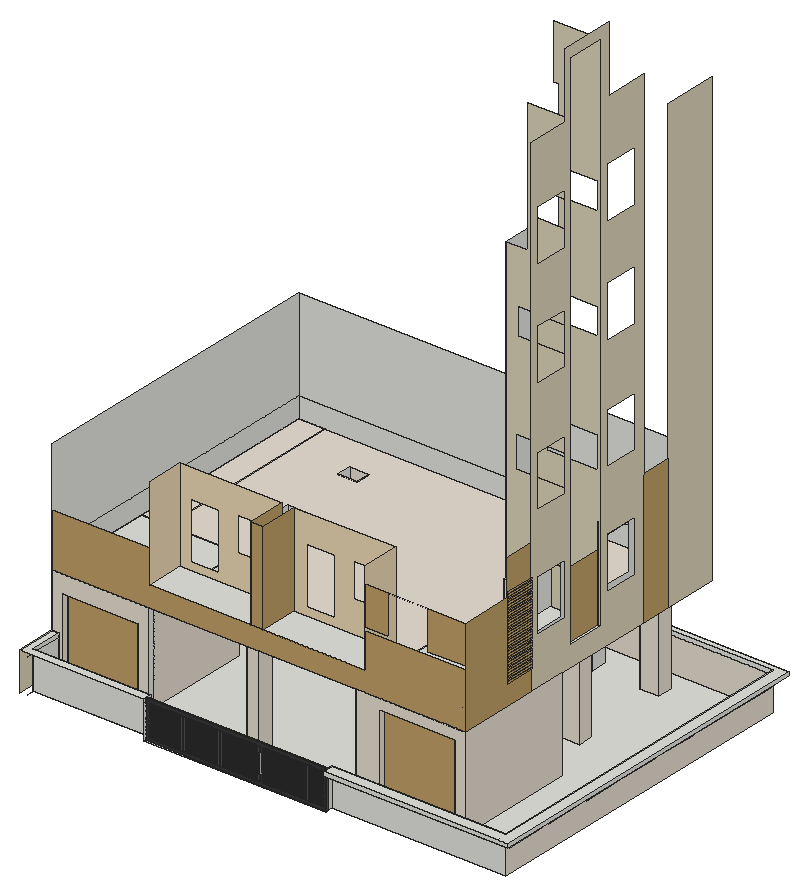
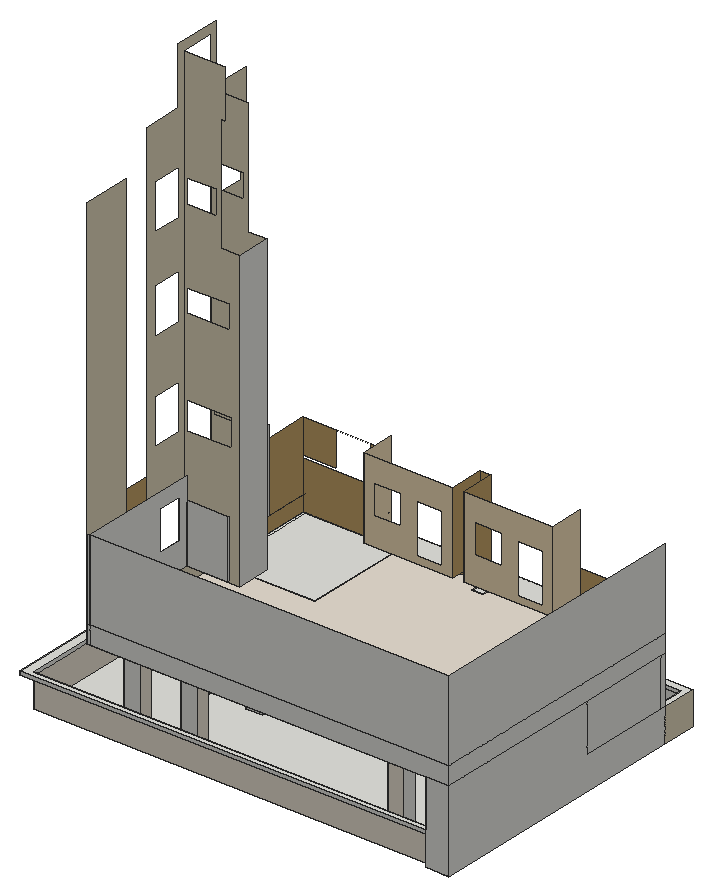
# SketchUp Ruby script. Lengths in inches.
U = 1.inch
M = Sketchup.active_model
def pt(a) = Geom::Point3d.new(a.map { |v| v * U })
def face(e, loops, mat)
  f = e.add_face(loops[0].map { |a| pt(a) })
  loops[1..].each { |l| e.add_face(l.map { |a| pt(a) }).erase! }
  f.material = f.back_material = mat if mat
  f
end
# faces: each face lists its corners as indices into pts; further lists are holes
def faces(e, pts, list, mat = nil) = list.each { |f| face(e, (f[0].is_a?(Array) ? f : [f]).map { |l| l.map { |i| pts[i] } }, mat) }
# xy, xz, yz: faces in a plane at the given z, y or x. An outline is a flat list of corners, or four numbers for a rectangle; further outlines are holes
def ring(l) = l.size == 4 ? [[l[0], l[1]], [l[2], l[1]], [l[2], l[3]], [l[0], l[3]]] : l.each_slice(2).to_a
def flat(e, list, mat, &to3) = list.each { |f| face(e, (f[0].is_a?(Array) ? f : [f]).map { |l| ring(l).map { |u, v| to3.(u, v) } }, mat) }
def xy(e, z, list, mat = nil) = flat(e, list, mat) { |x, y| [x, y, z] }
def xz(e, y, list, mat = nil) = flat(e, list, mat) { |x, z| [x, y, z] }
def yz(e, x, list, mat = nil) = flat(e, list, mat) { |y, z| [x, y, z] }
def lines(e, pts, list) = list.each { |a, b| e.add_line(pt(pts[a]), pt(pts[b])) }
# prism: a flat outline (further loops are holes) pulled along v
def prism(e, loops, v, mat = nil)
  f = face(e, loops, mat); d = Geom::Vector3d.new(v.map { |x| x * U })
  f.pushpull(f.normal.samedirection?(d) ? d.length : -d.length)
end
def box(e, o, s, mat = nil) = prism(e, [[o, [o[0] + s[0], o[1], o[2]], [o[0] + s[0], o[1] + s[1], o[2]], [o[0], o[1] + s[1], o[2]]]], [0, 0, s[2]], mat)
def at(x, y, z, deg = 0) = Geom::Transformation.translation(pt([x, y, z])) * Geom::Transformation.rotation(ORIGIN, Z_AXIS, deg.degrees)
def axes(o, x, y, z) = Geom::Transformation.new([*x, 0, *y, 0, *z, 0, *pt(o).to_a, 1])
def part(name) = M.definitions.add(name)
# library, detail: a bought-in or finely detailed component or shape, given as its bounding box
def library(name, o, s) = part(name).tap { |d| box(d.entities, o, s) }
def detail(e, o, s) = box(e.add_group.entities, o, s)
def put(e, d, t, mat = nil) = e.add_instance(d, t).tap { |i| i.material = mat if mat }
def group(e, t, mat = nil) = e.add_group.tap { |g| g.transformation = t; g.material = mat if mat }.entities
root = M.entities
M.materials.add("Generic").color = [191, 159, 103]
M.materials.add("Generic\#2").color = [235, 215, 180]
M.materials.add("Generic\#3").color = [218, 209, 183]
M.materials.add("Generic\#5").color = [230, 221, 208]
M.materials.add("[Color M02]").color = [198, 198, 198]
M.materials.add("[Color M06]").color = [86, 86, 86]
M.materials.add("[Color M07]").color = [58, 58, 58]
c1 = part("Group\#5")
xy(c1.entities,0,[[0,0,1,57.75]])
xy(c1.entities,2.57,[[0,0,1,57.75]])
xz(c1.entities,0,[[0,0,1,2.57]])
xz(c1.entities,57.75,[[0,0,1,2.57]])
yz(c1.entities,1,[[0,0,57.75,2.57]])
c2 = part("Group\#6")
put(c2.entities,c1,at(0,0,4.75))
put(c2.entities,c1,at(0,0,0))
put(c2.entities,c1,at(0,0,19))
put(c2.entities,c1,at(0,0,28.5))
put(c2.entities,c1,at(0,0,133))
put(c2.entities,c1,at(0,0,152))
put(c2.entities,c1,at(0,0,128.25))
put(c2.entities,c1,at(0,0,9.5))
put(c2.entities,c1,at(0,0,123.5))
put(c2.entities,c1,at(0,0,114))
put(c2.entities,c1,at(0,0,147.25))
put(c2.entities,c1,at(0,0,118.75))
put(c2.entities,c1,at(0,0,142.5))
put(c2.entities,c1,at(0,0,109.25))
put(c2.entities,c1,at(0,0,137.75))
put(c2.entities,c1,at(0,0,104.5))
put(c2.entities,c1,at(0,0,99.75))
put(c2.entities,c1,at(0,0,95))
put(c2.entities,c1,at(0,0,85.5))
put(c2.entities,c1,at(0,0,80.75))
put(c2.entities,c1,at(0,0,90.25))
put(c2.entities,c1,at(0,0,76))
put(c2.entities,c1,at(0,0,71.25))
put(c2.entities,c1,at(0,0,38))
put(c2.entities,c1,at(0,0,14.25))
put(c2.entities,c1,at(0,0,33.25))
put(c2.entities,c1,at(0,0,57))
put(c2.entities,c1,at(0,0,23.75))
put(c2.entities,c1,at(0,0,61.75))
put(c2.entities,c1,at(0,0,156.75))
put(c2.entities,c1,at(0,0,47.5))
put(c2.entities,c1,at(0,0,52.25))
put(c2.entities,c1,at(0,0,42.75))
put(c2.entities,c1,at(0,0,66.5))
xy(root,0,[[245.8125,5.75,599.47,21.4375],[[17.8125,21.4375,937.125,21.4375,937.125,671.4375,55.33,671.4375,55.33,683.8125,4.1875,683.8125,4.1875,83.8125,17.8125,83.8125],[596.08,83.8125,596.08,317.4375,809.375,317.4375,809.375,83.8125,787.75,83.8125,787.75,94.5625,641.71,94.5625,641.71,83.8125],[171.85,83.8125,193.48,301.3125],[17.8125,83.8125,25.82,301.3125],[159.02,434.88,196.46,463.32],[159.02,585.95,196.46,614.38],[613.85,411.28,651.29,439.72],[604.67,603.65,642.1,632.09],[731.98,603.65,769.42,632.09],[731.98,411.28,769.42,439.72],[382.78,83.8125,406.78,116.4375]],[17.8125,83.8125,25.82,94.5625],[171.85,83.8125,193.48,94.5625],[382.78,83.8125,406.78,116.4375],
  [596.08,83.8125,641.71,83.8125,641.71,94.5625,787.75,94.5625,787.75,83.8125,809.375,83.8125,809.375,317.4375,596.08,317.4375],[17.8125,94.5625,25.82,301.3125],[171.85,94.5625,193.48,301.3125]])
xy(root,59.89,[[950.0625,12.05,952.875,89.02],[950.0625,107.24,952.875,180.9],[950.0625,199.12,952.875,272.77],[950.0625,290.99,952.875,364.65],[950.0625,382.87,952.875,456.52],
  [950.0625,474.74,952.875,548.4],[950.0625,566.62,952.875,640.27]],"Generic")
xy(root,66.1875,[[599.47,0,952.875,5.75],[952.875,0,958.625,95.32],[937.125,5.75,937.125,671.4375,55.33,671.4375,55.33,683.8125,952.875,683.8125,952.875,5.75],[952.875,95.32,958.625,100.94],[952.875,100.94,958.625,187.19],
  [952.875,187.19,958.625,192.82],[952.875,192.82,958.625,279.07],[952.875,279.07,958.625,284.69],[952.875,284.69,958.625,370.94],[952.875,370.94,958.625,376.57],
  [952.875,376.57,958.625,462.82],[952.875,462.82,958.625,468.44],[952.875,468.44,958.625,554.69],[952.875,554.69,958.625,560.32],[952.875,560.32,958.625,646.57],
  [952.875,646.57,958.625,652.19],[952.875,652.19,958.625,683.8125]])
xy(root,74,[[599.47,0,958.625,0,958.625,683.8125,55.33,683.8125,55.33,671.4375,937.125,671.4375,937.125,21.4375,599.47,21.4375],[4.1875,5.75,245.8125,5.75,245.8125,21.4375,17.8125,21.4375,17.8125,83.8125,4.1875,83.8125],[4.1875,83.8125,17.8125,94.5625],[4.1875,94.5625,17.8125,301.3125]])
xy(root,144.62,[[25.82,94.5625,171.85,301.3125]])
xy(root,144.62,[[25.82,83.8125,171.85,94.5625]],"Generic\#5")
xy(root,158.37,[[641.71,83.8125,787.75,94.5625]],"Generic\#5")
xy(root,180,[[4.1875,83.8125,193.48,94.5625],[382.78,83.8125,406.78,116.4375],[596.08,83.8125,802.875,317.4375],[802.875,83.8125,809.375,317.4375],[4.1875,94.5625,193.48,301.3125]])
xy(root,180,[[[193.48,83.8125,193.48,301.3125,4.1875,301.3125,4.1875,683.8125,809.375,683.8125,809.375,317.4375,596.08,317.4375,596.08,83.8125,406.78,83.8125,406.78,116.4375,382.78,116.4375,382.78,83.8125],[604.67,603.65,642.1,632.09],[731.98,603.65,769.42,632.09],[613.85,411.28,651.29,439.72],[159.02,434.88,196.46,463.32],[159.02,585.95,196.46,614.38],[731.98,411.28,769.42,439.72]]],"Generic\#5")
xy(root,219.75,[[193.83,83.8125,391.53,158.75],[415.53,83.8125,613.23,158.75],[802.875,185.01,809.375,242.76],[684.5625,338.625,710.73,413.6875],[710.73,338.625,802.875,413.6875],
  [802.875,338.625,809.375,413.6875],[710.73,413.6875,802.875,414.4375]])
xz(root,0,[[599.47,66.1875,958.625,74]])
xz(root,21.4375,[[17.8125,0,245.8125,66.1875],[599.47,0,937.125,66.1875],[17.8125,66.1875,245.8125,74],[599.47,66.1875,937.125,74]])
xz(root,83.8125,[[4.1875,0,17.8125,74]])
xz(root,83.8125,[[4.1875,180,809.375,180,809.375,287.13,613.73,287.13,613.73,294.19,658.76,294.19,658.76,368.44,736.32,368.44,736.32,294.19,809.375,294.19,809.375,368.76,613.23,368.76,613.23,219.75,193.83,219.75,193.83,284.38,4.1875,284.38],[391.53,219.75,415.53,399.75]],"Generic")
xz(root,83.8125,[[17.8125,0,25.82,0,25.82,144.62,171.85,144.62,171.85,0,193.48,0,193.48,180,4.1875,180,4.1875,74,17.8125,74],[382.78,0,406.78,180],[596.08,0,641.71,0,641.71,158.37,787.75,158.37,787.75,0,809.375,0,809.375,180,596.08,180]],"Generic\#5")
xz(root,94.5625,[[17.8125,0,25.82,0,25.82,144.62,171.85,144.62,171.85,0,193.48,0,193.48,180,4.1875,180,4.1875,74,17.8125,74]])
xz(root,94.5625,[[25.82,0,171.85,144.62],[641.71,0,787.75,158.37]],"Generic")
xz(root,116.4375,[[382.78,0,406.78,180]])
xz(root,158.75,[[[193.83,219.75,391.53,399.75],[214.375,234.72,270.0625,344.97],[306.72,282.21,366.62,348.04]],[[415.53,219.75,613.23,399.75],[439.6875,234.72,495.375,344.97],[532.04,282.21,591.93,348.04]]],"Generic\#2")
xz(root,185.01,[[802.875,219.75,809.375,399.75]])
xz(root,301.3125,[[17.8125,0,17.8125,74,4.1875,74,4.1875,180,193.48,180,193.48,0,171.85,0,171.85,144.62,25.82,144.62,25.82,0]],"Generic\#5")
xz(root,317.4375,[[596.08,0,809.375,180]],"Generic\#5")
xz(root,338.625,[[684.5625,219.75,684.5625,879,726.91,879,726.91,1136.625,809.375,1136.625,809.375,219.75,802.875,219.75,802.875,993.42,736.34,993.42,736.34,941.3,802.875,941.3,802.875,774.4375,706.68,774.4375,706.68,722.9375,802.875,722.9375,802.875,549.89,703.98,549.89,703.98,488.89,802.875,488.89,802.875,350.51,710.73,350.51,710.73,219.75]],"Generic\#3")
xz(root,411.28,[[613.85,0,651.29,180],[731.98,0,769.42,180]],"Generic\#5")
xz(root,413.6875,[[684.5625,219.75,802.875,219.75,802.875,488.89,703.98,488.89,703.98,549.89,802.875,549.89,802.875,722.9375,706.68,722.9375,706.68,774.4375,802.875,774.4375,802.875,941.3,736.34,941.3,736.34,993.42,802.875,993.42,802.875,219.75,809.375,219.75,809.375,1243.75,718.29,1243.75,718.29,1136.625,726.91,1136.625,726.91,879,684.5625,879]],"Generic\#3")
xz(root,414.4375,[[710.73,219.75,802.875,350.51]])
xz(root,434.88,[[159.02,0,196.46,180]],"Generic\#5")
xz(root,439.72,[[613.85,0,651.29,180],[731.98,0,769.42,180]])
xz(root,463.32,[[159.02,0,196.46,180]])
xz(root,585.95,[[159.02,0,196.46,180]],"Generic\#5")
xz(root,603.65,[[604.67,0,642.1,180]])
xz(root,603.65,[[731.98,0,769.42,180]],"Generic\#5")
xz(root,614.38,[[159.02,0,196.46,180]],"Generic\#5")
xz(root,632.09,[[604.67,0,642.1,180],[731.98,0,769.42,180]])
xz(root,671.4375,[[55.33,66.1875,937.125,74]])
xz(root,671.4375,[[55.33,0,937.125,66.1875]],"Generic\#5")
xz(root,683.8125,[[4.1875,0,55.33,180],[55.33,66.1875,958.625,74],[4.1875,180,802.875,219.75],[802.875,180,809.375,219.75],[4.1875,219.75,802.875,399.75],
  [802.875,219.75,809.375,399.75]])
yz(root,4.1875,[[83.8125,0,83.8125,74,301.3125,74,301.3125,180,683.8125,180,683.8125,0],[83.8125,74,94.5625,180],[94.5625,74,301.3125,180],[83.8125,180,683.8125,219.75],[83.8125,219.75,683.8125,399.75]])
yz(root,4.1875,[[5.75,0,83.8125,74]],"Generic\#3")
yz(root,17.8125,[[21.4375,0,83.8125,66.1875],[83.8125,0,94.5625,66.1875],[94.5625,0,301.3125,66.1875],[21.4375,66.1875,83.8125,74],[83.8125,66.1875,94.5625,74],
  [94.5625,66.1875,301.3125,74]])
yz(root,25.82,[[83.8125,0,94.5625,144.62],[94.5625,0,301.3125,144.62]],"Generic\#5")
yz(root,55.33,[[317.4375,0,671.4375,0,671.4375,74,683.8125,74,683.8125,180,317.4375,180]],"Generic\#5")
yz(root,159.02,[[434.88,0,463.32,180],[585.95,0,614.38,180]])
yz(root,171.85,[[94.5625,0,301.3125,144.62]])
yz(root,171.85,[[83.8125,0,94.5625,144.62]],"Generic\#5")
yz(root,193.48,[[83.8125,0,94.5625,180]])
yz(root,193.48,[[94.5625,0,301.3125,180]],"Generic\#5")
yz(root,193.83,[[[83.8125,219.75,158.75,399.75],[90.04,254.33,89.73,254.375,89.44,254.49,89.2,254.68,89.01,254.93,88.89,255.21,88.85,255.52,88.89,255.83,89.01,256.11,89.2,256.36,89.44,256.55,89.73,256.67,90.04,256.71,90.35,256.67,90.63,256.55,90.88,256.36,91.07,256.11,91.18,255.83,91.23,255.52,91.18,255.21,91.07,254.93,90.88,254.68,90.63,254.49,90.35,254.375],[90.04,247.77,89.73,247.8125,89.44,247.93,89.2,248.12,89.01,248.36,88.89,248.65,88.85,248.96,88.89,249.27,89.01,249.55,89.2,249.8,89.44,249.99,89.73,250.11,90.04,250.15,90.35,250.11,90.63,249.99,90.88,249.8,91.07,249.55,91.18,249.27,91.23,248.96,91.18,248.65,91.07,248.36,90.88,248.12,90.63,247.93,90.35,247.8125],[90.04,240.77,89.73,240.8125,89.44,240.93,89.2,241.12,89.01,241.36,88.89,241.65,88.85,241.96,88.89,242.27,89.01,242.55,89.2,242.8,89.44,242.99,89.73,243.11,90.04,243.15,90.35,243.11,90.63,242.99,90.88,242.8,91.07,242.55,91.18,242.27,91.23,241.96,91.18,241.65,91.07,241.36,90.88,241.12,90.63,240.93,90.35,240.8125],[90.04,233.77,89.73,233.8125,89.44,233.93,89.2,234.12,89.01,234.36,88.89,234.65,88.85,234.96,88.89,235.27,89.01,235.55,89.2,235.8,89.44,235.99,89.73,236.11,90.04,236.15,90.35,236.11,90.63,235.99,90.88,235.8,91.07,235.55,91.18,235.27,91.23,234.96,91.18,234.65,91.07,234.36,90.88,234.12,90.63,233.93,90.35,233.8125],[90.04,227.08,89.73,227.125,89.44,227.24,89.2,227.43,89.01,227.68,88.89,227.96,88.85,228.27,88.89,228.58,89.01,228.86,89.2,229.11,89.44,229.3,89.73,229.42,90.04,229.46,90.35,229.42,90.63,229.3,90.88,229.11,91.07,228.86,91.18,228.58,91.23,228.27,91.18,227.96,91.07,227.68,90.88,227.43,90.63,227.24,90.35,227.125]]],"Generic\#2")
yz(root,196.46,[[434.88,0,463.32,180],[585.95,0,614.38,180]],"Generic\#5")
yz(root,245.8125,[[5.75,0,21.4375,66.1875],[5.75,66.1875,21.4375,74]])
yz(root,382.78,[[83.8125,0,116.4375,180]],"Generic\#5")
yz(root,391.53,[[[83.8125,219.75,158.75,399.75],[90.04,227.08,90.35,227.125,90.63,227.24,90.88,227.43,91.07,227.68,91.18,227.96,91.23,228.27,91.18,228.58,91.07,228.86,90.88,229.11,90.63,229.3,90.35,229.42,90.04,229.46,89.73,229.42,89.44,229.3,89.2,229.11,89.01,228.86,88.89,228.58,88.85,228.27,88.89,227.96,89.01,227.68,89.2,227.43,89.44,227.24,89.73,227.125],[90.04,233.77,90.35,233.8125,90.63,233.93,90.88,234.12,91.07,234.36,91.18,234.65,91.23,234.96,91.18,235.27,91.07,235.55,90.88,235.8,90.63,235.99,90.35,236.11,90.04,236.15,89.73,236.11,89.44,235.99,89.2,235.8,89.01,235.55,88.89,235.27,88.85,234.96,88.89,234.65,89.01,234.36,89.2,234.12,89.44,233.93,89.73,233.8125],[90.04,240.77,90.35,240.8125,90.63,240.93,90.88,241.12,91.07,241.36,91.18,241.65,91.23,241.96,91.18,242.27,91.07,242.55,90.88,242.8,90.63,242.99,90.35,243.11,90.04,243.15,89.73,243.11,89.44,242.99,89.2,242.8,89.01,242.55,88.89,242.27,88.85,241.96,88.89,241.65,89.01,241.36,89.2,241.12,89.44,240.93,89.73,240.8125],[90.04,247.77,90.35,247.8125,90.63,247.93,90.88,248.12,91.07,248.36,91.18,248.65,91.23,248.96,91.18,249.27,91.07,249.55,90.88,249.8,90.63,249.99,90.35,250.11,90.04,250.15,89.73,250.11,89.44,249.99,89.2,249.8,89.01,249.55,88.89,249.27,88.85,248.96,88.89,248.65,89.01,248.36,89.2,248.12,89.44,247.93,89.73,247.8125],[90.04,254.33,90.35,254.375,90.63,254.49,90.88,254.68,91.07,254.93,91.18,255.21,91.23,255.52,91.18,255.83,91.07,256.11,90.88,256.36,90.63,256.55,90.35,256.67,90.04,256.71,89.73,256.67,89.44,256.55,89.2,256.36,89.01,256.11,88.89,255.83,88.85,255.52,88.89,255.21,89.01,254.93,89.2,254.68,89.44,254.49,89.73,254.375]]],"Generic")
yz(root,406.78,[[83.8125,0,116.4375,180]],"Generic\#5")
yz(root,415.53,[[[83.8125,219.75,158.75,399.75],[89.21,233.84,89.0625,233.86,88.93,233.91,88.8125,234,88.72,234.12,88.67,234.25,88.65,234.4,88.67,234.54,88.72,234.68,88.8125,234.8,88.93,234.89,89.0625,234.94,89.21,234.96,89.36,234.94,89.49,234.89,89.61,234.8,89.7,234.68,89.75,234.54,89.77,234.4,89.75,234.25,89.7,234.12,89.61,234,89.49,233.91,89.36,233.86],[89.21,241.34,89.0625,241.36,88.93,241.41,88.8125,241.5,88.72,241.62,88.67,241.75,88.65,241.9,88.67,242.04,88.72,242.18,88.8125,242.3,88.93,242.39,89.0625,242.44,89.21,242.46,89.36,242.44,89.49,242.39,89.61,242.3,89.7,242.18,89.75,242.04,89.77,241.9,89.75,241.75,89.7,241.62,89.61,241.5,89.49,241.41,89.36,241.36],[89.21,226.46,89.0625,226.48,88.93,226.54,88.8125,226.625,88.72,226.74,88.67,226.88,88.65,227.02,88.67,227.17,88.72,227.31,88.8125,227.42,88.93,227.51,89.0625,227.57,89.21,227.59,89.36,227.57,89.49,227.51,89.61,227.42,89.7,227.31,89.75,227.17,89.77,227.02,89.75,226.88,89.7,226.74,89.61,226.625,89.49,226.54,89.36,226.48],[89.21,256.27,89.0625,256.29,88.93,256.35,88.8125,256.4375,88.72,256.56,88.67,256.69,88.65,256.84,88.67,256.98,88.72,257.12,88.8125,257.23,88.93,257.32,89.0625,257.38,89.21,257.4,89.36,257.38,89.49,257.32,89.61,257.23,89.7,257.12,89.75,256.98,89.77,256.84,89.75,256.69,89.7,256.56,89.61,256.4375,89.49,256.35,89.36,256.29],[89.21,248.84,89.0625,248.86,88.93,248.91,88.8125,249,88.72,249.12,88.67,249.25,88.65,249.4,88.67,249.54,88.72,249.68,88.8125,249.8,88.93,249.89,89.0625,249.94,89.21,249.96,89.36,249.94,89.49,249.89,89.61,249.8,89.7,249.68,89.75,249.54,89.77,249.4,89.75,249.25,89.7,249.12,89.61,249,89.49,248.91,89.36,248.86]]],"Generic")
yz(root,596.08,[[83.8125,0,317.4375,180]],"Generic\#5")
yz(root,599.47,[[5.75,0,21.4375,66.1875],[0,66.1875,5.75,74],[5.75,66.1875,21.4375,74]])
yz(root,604.67,[[603.65,0,632.09,180]],"Generic\#5")
yz(root,613.23,[[[83.8125,219.75,158.75,399.75],[89.21,226.46,89.36,226.48,89.49,226.54,89.61,226.625,89.7,226.74,89.75,226.88,89.77,227.02,89.75,227.17,89.7,227.31,89.61,227.42,89.49,227.51,89.36,227.57,89.21,227.59,89.0625,227.57,88.93,227.51,88.8125,227.42,88.72,227.31,88.67,227.17,88.65,227.02,88.67,226.88,88.72,226.74,88.8125,226.625,88.93,226.54,89.0625,226.48],[89.21,233.84,89.36,233.86,89.49,233.91,89.61,234,89.7,234.12,89.75,234.25,89.77,234.4,89.75,234.54,89.7,234.68,89.61,234.8,89.49,234.89,89.36,234.94,89.21,234.96,89.0625,234.94,88.93,234.89,88.8125,234.8,88.72,234.68,88.67,234.54,88.65,234.4,88.67,234.25,88.72,234.12,88.8125,234,88.93,233.91,89.0625,233.86],[89.21,241.34,89.36,241.36,89.49,241.41,89.61,241.5,89.7,241.62,89.75,241.75,89.77,241.9,89.75,242.04,89.7,242.18,89.61,242.3,89.49,242.39,89.36,242.44,89.21,242.46,89.0625,242.44,88.93,242.39,88.8125,242.3,88.72,242.18,88.67,242.04,88.65,241.9,88.67,241.75,88.72,241.62,88.8125,241.5,88.93,241.41,89.0625,241.36],[89.21,248.84,89.36,248.86,89.49,248.91,89.61,249,89.7,249.12,89.75,249.25,89.77,249.4,89.75,249.54,89.7,249.68,89.61,249.8,89.49,249.89,89.36,249.94,89.21,249.96,89.0625,249.94,88.93,249.89,88.8125,249.8,88.72,249.68,88.67,249.54,88.65,249.4,88.67,249.25,88.72,249.12,88.8125,249,88.93,248.91,89.0625,248.86],[89.21,256.27,89.36,256.29,89.49,256.35,89.61,256.4375,89.7,256.56,89.75,256.69,89.77,256.84,89.75,256.98,89.7,257.12,89.61,257.23,89.49,257.32,89.36,257.38,89.21,257.4,89.0625,257.38,88.93,257.32,88.8125,257.23,88.72,257.12,88.67,256.98,88.65,256.84,88.67,256.69,88.72,256.56,88.8125,256.4375,88.93,256.35,89.0625,256.29]]],"Generic\#2")
yz(root,613.85,[[411.28,0,439.72,180]],"Generic\#5")
yz(root,641.71,[[83.8125,0,94.5625,158.37]],"Generic\#5")
yz(root,642.1,[[603.65,0,632.09,180]])
yz(root,651.29,[[411.28,0,439.72,180]],"Generic\#5")
yz(root,684.5625,[[338.625,219.75,413.6875,879]])
yz(root,710.73,[[338.625,219.75,414.4375,350.51]])
yz(root,731.98,[[411.28,0,439.72,180]])
yz(root,731.98,[[603.65,0,632.09,180]],"Generic\#5")
yz(root,769.42,[[411.28,0,439.72,180],[603.65,0,632.09,180]],"Generic\#5")
yz(root,787.75,[[83.8125,0,94.5625,158.37]],"Generic\#5")
yz(root,802.875,[[185.01,219.75,242.76,399.75],[[242.76,219.75,338.625,399.75],[257.24,272.84,324.36,373.53]],[413.6875,219.75,414.4375,350.51],[[414.4375,219.75,414.4375,350.51,413.6875,350.51,413.6875,399.75,683.8125,399.75,683.8125,219.75],[434.88,279.25,489.19,367.13]]])
yz(root,802.875,[[338.625,219.75,413.6875,350.51]],"Generic")
yz(root,809.375,[[83.8125,180,242.76,180,242.76,219.75,185.01,219.75,185.01,368.76,83.8125,368.76],[518.09,180,575.84,439.5],[185.01,219.75,242.76,439.5]],"Generic")
yz(root,809.375,[[[242.76,180,518.09,180,518.09,1136.625,431.25,1136.625,431.25,1265.4375,325.3125,1265.4375,325.3125,1136.625,338.625,1136.625,338.625,1243.75,413.6875,1243.75,413.6875,219.75,338.625,219.75,338.625,1136.625,242.76,1136.625],[428.47,272.84,495.59,373.53],[428.47,489.97,495.59,590.66],[428.47,710.22,495.59,810.91],[428.47,918.09,495.59,1018.78],[257.24,710.22,324.36,810.91],[257.24,918.09,324.36,1018.78],[257.24,489.97,324.36,590.66],[257.24,272.84,324.36,373.53]],[575.84,180,683.8125,1059]],"Generic\#3")
yz(root,809.375,[[83.8125,0,317.4375,180]],"Generic\#5")
yz(root,937.125,[[21.4375,66.1875,671.4375,74]])
yz(root,937.125,[[21.4375,0,671.4375,66.1875]],"Generic\#5")
yz(root,958.625,[[0,66.1875,683.8125,74]])
p = [[802.875,83.8125,219.75],[802.875,185.01,219.75],[17.8125,21.4375,0],[17.8125,5.75,0],[17.8125,21.4375,66.1875],[17.8125,5.75,66.1875],
  [937.125,5.75,66.1875],[937.125,5.75,74]]
lines(root,p,[[0,1],[2,3],[4,5],[6,7]])
g1 = group(root,at(245.8125,5.75,0))
xy(g1,0,[[0,3.41,353.66,6.41]],"[Color M06]")
xy(g1,5.95,[[9.7,3.41,11.95,6.41],[15.7,3.41,17.95,6.41],[21.7,3.41,23.95,6.41],[27.7,3.41,29.95,6.41],[33.7,3.41,35.95,6.41],
  [39.7,3.41,41.95,6.41],[45.7,3.41,47.95,6.41],[51.7,3.41,53.95,6.41],[57.7,3.41,59.95,6.41],[63.7,3.41,65.95,6.41],
  [69.7,3.41,71.95,6.41],[75.7,3.41,77.95,6.41],[81.7,3.41,83.95,6.41],[87.7,3.41,89.95,6.41],[93.7,3.41,95.95,6.41],
  [99.7,3.41,101.95,6.41],[105.7,3.41,107.95,6.41],[111.7,3.41,113.95,6.41],[117.7,3.41,119.95,6.41],[123.7,3.41,125.95,6.41],
  [129.7,3.41,131.95,6.41],[135.7,3.41,137.95,6.41],[141.7,3.41,143.95,6.41],[147.7,3.41,149.95,6.41],[153.7,3.41,155.95,6.41],
  [159.7,3.41,161.95,6.41],[165.7,3.41,167.95,6.41],[171.7,3.41,173.95,6.41],[177.7,3.41,179.95,6.41],[183.7,3.41,185.95,6.41],
  [189.7,3.41,191.95,6.41],[195.7,3.41,197.95,6.41],[201.7,3.41,203.95,6.41],[207.7,3.41,209.95,6.41],[213.7,3.41,215.95,6.41],
  [219.7,3.41,221.95,6.41],[227.95,3.41,230.26,6.41],[233.67,3.41,235.7,6.41],[239.1,3.41,241.14,6.41],[244.54,3.41,246.58,6.41],
  [249.98,3.41,252.01,6.41],[255.42,3.41,257.45,6.41],[260.85,3.41,262.89,6.41],[266.29,3.41,268.33,6.41],[271.73,3.41,273.76,6.41],
  [277.17,3.41,279.2,6.41],[282.6,3.41,284.64,6.41],[288.04,3.41,290.08,6.41],[293.48,3.41,295.51,6.41],[298.92,3.41,300.95,6.41],
  [304.35,3.41,306.39,6.41],[309.79,3.41,311.83,6.41],[315.23,3.41,317.26,6.41],[320.67,3.41,322.7,6.41],[326.1,3.41,328.14,6.41],
  [331.54,3.41,333.58,6.41],[336.98,3.41,339.01,6.41],[342.42,3.41,344.45,6.41]],"[Color M06]")
xy(g1,20.68,[[223.11,0,225.86,3.41]],"[Color M02]")
xy(g1,21.99,[[223.11,1.3125,225.86,3.41]],"[Color M02]")
xy(g1,56.82,[[223.11,1.3125,225.86,3.41]],"[Color M06]")
xy(g1,58.13,[[223.11,0,225.86,3.41]],"[Color M02]")
xy(g1,68.05,[[9.7,3.41,11.95,6.41],[15.7,3.41,17.95,6.41],[21.7,3.41,23.95,6.41],[27.7,3.41,29.95,6.41],[33.7,3.41,35.95,6.41],
  [39.7,3.41,41.95,6.41],[45.7,3.41,47.95,6.41],[51.7,3.41,53.95,6.41],[57.7,3.41,59.95,6.41],[63.7,3.41,65.95,6.41],
  [69.7,3.41,71.95,6.41],[75.7,3.41,77.95,6.41],[81.7,3.41,83.95,6.41],[87.7,3.41,89.95,6.41],[93.7,3.41,95.95,6.41],
  [99.7,3.41,101.95,6.41],[105.7,3.41,107.95,6.41],[111.7,3.41,113.95,6.41],[117.7,3.41,119.95,6.41],[123.7,3.41,125.95,6.41],
  [129.7,3.41,131.95,6.41],[135.7,3.41,137.95,6.41],[141.7,3.41,143.95,6.41],[147.7,3.41,149.95,6.41],[153.7,3.41,155.95,6.41],
  [159.7,3.41,161.95,6.41],[165.7,3.41,167.95,6.41],[171.7,3.41,173.95,6.41],[177.7,3.41,179.95,6.41],[183.7,3.41,185.95,6.41],
  [189.7,3.41,191.95,6.41],[195.7,3.41,197.95,6.41],[201.7,3.41,203.95,6.41],[207.7,3.41,209.95,6.41],[213.7,3.41,215.95,6.41],
  [219.7,3.41,221.95,6.41],[227.95,3.41,230.26,6.41],[233.67,3.41,235.7,6.41],[239.1,3.41,241.14,6.41],[244.54,3.41,246.58,6.41],
  [249.98,3.41,252.01,6.41],[255.42,3.41,257.45,6.41],[260.85,3.41,262.89,6.41],[266.29,3.41,268.33,6.41],[271.73,3.41,273.76,6.41],
  [277.17,3.41,279.2,6.41],[282.6,3.41,284.64,6.41],[288.04,3.41,290.08,6.41],[293.48,3.41,295.51,6.41],[298.92,3.41,300.95,6.41],
  [304.35,3.41,306.39,6.41],[309.79,3.41,311.83,6.41],[315.23,3.41,317.26,6.41],[320.67,3.41,322.7,6.41],[326.1,3.41,328.14,6.41],
  [331.54,3.41,333.58,6.41],[336.98,3.41,339.01,6.41],[342.42,3.41,344.45,6.41]],"[Color M06]")
xy(g1,74,[[0,3.41,353.66,6.41]],"[Color M06]")
xz(g1,0,[[223.11,20.68,225.86,58.13]],"[Color M02]")
xz(g1,1.3125,[[223.11,21.99,225.86,56.82]],"[Color M06]")
xz(g1,3.41,[[5.95,5.95,9.7,68.05],[11.95,5.95,15.7,68.05],[17.95,5.95,21.7,68.05],[23.95,5.95,27.7,68.05],[29.95,5.95,33.7,68.05],
  [35.95,5.95,39.7,68.05],[41.95,5.95,45.7,68.05],[47.95,5.95,51.7,68.05],[53.95,5.95,57.7,68.05],[59.95,5.95,63.7,68.05],
  [65.95,5.95,69.7,68.05],[71.95,5.95,75.7,68.05],[77.95,5.95,81.7,68.05],[83.95,5.95,87.7,68.05],[89.95,5.95,93.7,68.05],
  [95.95,5.95,99.7,68.05],[101.95,5.95,105.7,68.05],[107.95,5.95,111.7,68.05],[113.95,5.95,117.7,68.05],[119.95,5.95,123.7,68.05],
  [125.95,5.95,129.7,68.05],[131.95,5.95,135.7,68.05],[137.95,5.95,141.7,68.05],[143.95,5.95,147.7,68.05],[149.95,5.95,153.7,68.05],
  [155.95,5.95,159.7,68.05],[161.95,5.95,165.7,68.05],[167.95,5.95,171.7,68.05],[173.95,5.95,177.7,68.05],[179.95,5.95,183.7,68.05],
  [185.95,5.95,189.7,68.05],[191.95,5.95,195.7,68.05],[197.95,5.95,201.7,68.05],[203.95,5.95,207.7,68.05],[209.95,5.95,213.7,68.05],
  [215.95,5.95,219.7,68.05],[230.26,5.95,233.67,68.05],[235.7,5.95,239.1,68.05],[241.14,5.95,244.54,68.05],[246.58,5.95,249.98,68.05],
  [252.01,5.95,255.42,68.05],[257.45,5.95,260.85,68.05],[262.89,5.95,266.29,68.05],[268.33,5.95,271.73,68.05],[273.76,5.95,277.17,68.05],
  [279.2,5.95,282.6,68.05],[284.64,5.95,288.04,68.05],[290.08,5.95,293.48,68.05],[295.51,5.95,298.92,68.05],[300.95,5.95,304.35,68.05],
  [306.39,5.95,309.79,68.05],[311.83,5.95,315.23,68.05],[317.26,5.95,320.67,68.05],[322.7,5.95,326.1,68.05],[328.14,5.95,331.54,68.05],
  [333.58,5.95,336.98,68.05],[339.01,5.95,342.42,68.05],[344.45,5.95,347.71,68.05],[223.11,56.82,225.86,58.13]],"[Color M06]")
xz(g1,3.41,[[[0,0,353.66,74],[5.95,5.95,221.95,68.05],[227.95,5.95,347.71,68.05],[223.11,56.82,225.86,58.13],[223.11,20.68,225.86,21.99]]],"[Color M07]")
xz(g1,6.41,[[[0,0,353.66,74],[227.95,5.95,230.26,68.05],[219.7,5.95,221.95,68.05],[213.7,5.95,215.95,68.05],[207.7,5.95,209.95,68.05],[201.7,5.95,203.95,68.05],[195.7,5.95,197.95,68.05],[189.7,5.95,191.95,68.05],[183.7,5.95,185.95,68.05],[177.7,5.95,179.95,68.05],[171.7,5.95,173.95,68.05],[165.7,5.95,167.95,68.05],[159.7,5.95,161.95,68.05],[153.7,5.95,155.95,68.05],[147.7,5.95,149.95,68.05],[141.7,5.95,143.95,68.05],[135.7,5.95,137.95,68.05],[129.7,5.95,131.95,68.05],[123.7,5.95,125.95,68.05],[117.7,5.95,119.95,68.05],[111.7,5.95,113.95,68.05],[105.7,5.95,107.95,68.05],[99.7,5.95,101.95,68.05],[93.7,5.95,95.95,68.05],[87.7,5.95,89.95,68.05],[81.7,5.95,83.95,68.05],[75.7,5.95,77.95,68.05],[69.7,5.95,71.95,68.05],[63.7,5.95,65.95,68.05],[57.7,5.95,59.95,68.05],[51.7,5.95,53.95,68.05],[45.7,5.95,47.95,68.05],[39.7,5.95,41.95,68.05],[33.7,5.95,35.95,68.05],[27.7,5.95,29.95,68.05],[21.7,5.95,23.95,68.05],[15.7,5.95,17.95,68.05],[9.7,5.95,11.95,68.05],[239.1,5.95,241.14,68.05],[244.54,5.95,246.58,68.05],[249.98,5.95,252.01,68.05],[255.42,5.95,257.45,68.05],[260.85,5.95,262.89,68.05],[266.29,5.95,268.33,68.05],[271.73,5.95,273.76,68.05],[277.17,5.95,279.2,68.05],[282.6,5.95,284.64,68.05],[288.04,5.95,290.08,68.05],[293.48,5.95,295.51,68.05],[298.92,5.95,300.95,68.05],[304.35,5.95,306.39,68.05],[309.79,5.95,311.83,68.05],[315.23,5.95,317.26,68.05],[320.67,5.95,322.7,68.05],[326.1,5.95,328.14,68.05],[331.54,5.95,333.58,68.05],[336.98,5.95,339.01,68.05],[342.42,5.95,344.45,68.05],[233.67,5.95,235.7,68.05]]],"[Color M06]")
yz(g1,0,[[3.41,0,6.41,74]],"[Color M06]")
yz(g1,9.7,[[3.41,5.95,6.41,68.05]],"[Color M06]")
yz(g1,11.95,[[3.41,5.95,6.41,68.05]],"[Color M06]")
yz(g1,15.7,[[3.41,5.95,6.41,68.05]],"[Color M06]")
yz(g1,17.95,[[3.41,5.95,6.41,68.05]],"[Color M06]")
yz(g1,21.7,[[3.41,5.95,6.41,68.05]],"[Color M06]")
yz(g1,23.95,[[3.41,5.95,6.41,68.05]],"[Color M06]")
yz(g1,27.7,[[3.41,5.95,6.41,68.05]],"[Color M06]")
yz(g1,29.95,[[3.41,5.95,6.41,68.05]],"[Color M06]")
yz(g1,33.7,[[3.41,5.95,6.41,68.05]],"[Color M06]")
yz(g1,35.95,[[3.41,5.95,6.41,68.05]],"[Color M06]")
yz(g1,39.7,[[3.41,5.95,6.41,68.05]],"[Color M06]")
yz(g1,41.95,[[3.41,5.95,6.41,68.05]],"[Color M06]")
yz(g1,45.7,[[3.41,5.95,6.41,68.05]],"[Color M06]")
yz(g1,47.95,[[3.41,5.95,6.41,68.05]],"[Color M06]")
yz(g1,51.7,[[3.41,5.95,6.41,68.05]],"[Color M06]")
yz(g1,53.95,[[3.41,5.95,6.41,68.05]],"[Color M06]")
yz(g1,57.7,[[3.41,5.95,6.41,68.05]],"[Color M06]")
yz(g1,59.95,[[3.41,5.95,6.41,68.05]],"[Color M06]")
yz(g1,63.7,[[3.41,5.95,6.41,68.05]],"[Color M06]")
yz(g1,65.95,[[3.41,5.95,6.41,68.05]],"[Color M06]")
yz(g1,69.7,[[3.41,5.95,6.41,68.05]],"[Color M06]")
yz(g1,71.95,[[3.41,5.95,6.41,68.05]],"[Color M06]")
yz(g1,75.7,[[3.41,5.95,6.41,68.05]],"[Color M06]")
yz(g1,77.95,[[3.41,5.95,6.41,68.05]],"[Color M06]")
yz(g1,81.7,[[3.41,5.95,6.41,68.05]],"[Color M06]")
yz(g1,83.95,[[3.41,5.95,6.41,68.05]],"[Color M06]")
yz(g1,87.7,[[3.41,5.95,6.41,68.05]],"[Color M06]")
yz(g1,89.95,[[3.41,5.95,6.41,68.05]],"[Color M06]")
yz(g1,93.7,[[3.41,5.95,6.41,68.05]],"[Color M06]")
yz(g1,95.95,[[3.41,5.95,6.41,68.05]],"[Color M06]")
yz(g1,99.7,[[3.41,5.95,6.41,68.05]],"[Color M06]")
yz(g1,101.95,[[3.41,5.95,6.41,68.05]],"[Color M06]")
yz(g1,105.7,[[3.41,5.95,6.41,68.05]],"[Color M06]")
yz(g1,107.95,[[3.41,5.95,6.41,68.05]],"[Color M06]")
yz(g1,111.7,[[3.41,5.95,6.41,68.05]],"[Color M06]")
yz(g1,113.95,[[3.41,5.95,6.41,68.05]],"[Color M06]")
yz(g1,117.7,[[3.41,5.95,6.41,68.05]],"[Color M06]")
yz(g1,119.95,[[3.41,5.95,6.41,68.05]],"[Color M06]")
yz(g1,123.7,[[3.41,5.95,6.41,68.05]],"[Color M06]")
yz(g1,125.95,[[3.41,5.95,6.41,68.05]],"[Color M06]")
yz(g1,129.7,[[3.41,5.95,6.41,68.05]],"[Color M06]")
yz(g1,131.95,[[3.41,5.95,6.41,68.05]],"[Color M06]")
yz(g1,135.7,[[3.41,5.95,6.41,68.05]],"[Color M06]")
yz(g1,137.95,[[3.41,5.95,6.41,68.05]],"[Color M06]")
yz(g1,141.7,[[3.41,5.95,6.41,68.05]],"[Color M06]")
yz(g1,143.95,[[3.41,5.95,6.41,68.05]],"[Color M06]")
yz(g1,147.7,[[3.41,5.95,6.41,68.05]],"[Color M06]")
yz(g1,149.95,[[3.41,5.95,6.41,68.05]],"[Color M06]")
yz(g1,153.7,[[3.41,5.95,6.41,68.05]],"[Color M06]")
yz(g1,155.95,[[3.41,5.95,6.41,68.05]],"[Color M06]")
yz(g1,159.7,[[3.41,5.95,6.41,68.05]],"[Color M06]")
yz(g1,161.95,[[3.41,5.95,6.41,68.05]],"[Color M06]")
yz(g1,165.7,[[3.41,5.95,6.41,68.05]],"[Color M06]")
yz(g1,167.95,[[3.41,5.95,6.41,68.05]],"[Color M06]")
yz(g1,171.7,[[3.41,5.95,6.41,68.05]],"[Color M06]")
yz(g1,173.95,[[3.41,5.95,6.41,68.05]],"[Color M06]")
yz(g1,177.7,[[3.41,5.95,6.41,68.05]],"[Color M06]")
yz(g1,179.95,[[3.41,5.95,6.41,68.05]],"[Color M06]")
yz(g1,183.7,[[3.41,5.95,6.41,68.05]],"[Color M06]")
yz(g1,185.95,[[3.41,5.95,6.41,68.05]],"[Color M06]")
yz(g1,189.7,[[3.41,5.95,6.41,68.05]],"[Color M06]")
yz(g1,191.95,[[3.41,5.95,6.41,68.05]],"[Color M06]")
yz(g1,195.7,[[3.41,5.95,6.41,68.05]],"[Color M06]")
yz(g1,197.95,[[3.41,5.95,6.41,68.05]],"[Color M06]")
yz(g1,201.7,[[3.41,5.95,6.41,68.05]],"[Color M06]")
yz(g1,203.95,[[3.41,5.95,6.41,68.05]],"[Color M06]")
yz(g1,207.7,[[3.41,5.95,6.41,68.05]],"[Color M06]")
yz(g1,209.95,[[3.41,5.95,6.41,68.05]],"[Color M06]")
yz(g1,213.7,[[3.41,5.95,6.41,68.05]],"[Color M06]")
yz(g1,215.95,[[3.41,5.95,6.41,68.05]],"[Color M06]")
yz(g1,219.7,[[3.41,5.95,6.41,68.05]],"[Color M06]")
yz(g1,221.95,[[3.41,5.95,6.41,68.05]],"[Color M06]")
yz(g1,223.11,[[0,20.68,0,58.13,3.41,58.13,3.41,56.82,1.3125,56.82,1.3125,21.99,3.41,21.99,3.41,20.68]],"[Color M02]")
yz(g1,225.86,[[0,20.68,3.41,20.68,3.41,21.99,1.3125,21.99,1.3125,56.82,3.41,56.82,3.41,58.13,0,58.13]],"[Color M02]")
yz(g1,227.95,[[3.41,5.95,6.41,68.05]],"[Color M06]")
yz(g1,230.26,[[3.41,5.95,6.41,68.05]],"[Color M06]")
yz(g1,233.67,[[3.41,5.95,6.41,68.05]],"[Color M06]")
yz(g1,235.7,[[3.41,5.95,6.41,68.05]],"[Color M06]")
yz(g1,239.1,[[3.41,5.95,6.41,68.05]],"[Color M06]")
yz(g1,241.14,[[3.41,5.95,6.41,68.05]],"[Color M06]")
yz(g1,244.54,[[3.41,5.95,6.41,68.05]],"[Color M06]")
yz(g1,246.58,[[3.41,5.95,6.41,68.05]],"[Color M06]")
yz(g1,249.98,[[3.41,5.95,6.41,68.05]],"[Color M06]")
yz(g1,252.01,[[3.41,5.95,6.41,68.05]],"[Color M06]")
yz(g1,255.42,[[3.41,5.95,6.41,68.05]],"[Color M06]")
yz(g1,257.45,[[3.41,5.95,6.41,68.05]],"[Color M06]")
yz(g1,260.85,[[3.41,5.95,6.41,68.05]],"[Color M06]")
yz(g1,262.89,[[3.41,5.95,6.41,68.05]],"[Color M06]")
yz(g1,266.29,[[3.41,5.95,6.41,68.05]],"[Color M06]")
yz(g1,268.33,[[3.41,5.95,6.41,68.05]],"[Color M06]")
yz(g1,271.73,[[3.41,5.95,6.41,68.05]],"[Color M06]")
yz(g1,273.76,[[3.41,5.95,6.41,68.05]],"[Color M06]")
yz(g1,277.17,[[3.41,5.95,6.41,68.05]],"[Color M06]")
yz(g1,279.2,[[3.41,5.95,6.41,68.05]],"[Color M06]")
yz(g1,282.6,[[3.41,5.95,6.41,68.05]],"[Color M06]")
yz(g1,284.64,[[3.41,5.95,6.41,68.05]],"[Color M06]")
yz(g1,288.04,[[3.41,5.95,6.41,68.05]],"[Color M06]")
yz(g1,290.08,[[3.41,5.95,6.41,68.05]],"[Color M06]")
yz(g1,293.48,[[3.41,5.95,6.41,68.05]],"[Color M06]")
yz(g1,295.51,[[3.41,5.95,6.41,68.05]],"[Color M06]")
yz(g1,298.92,[[3.41,5.95,6.41,68.05]],"[Color M06]")
yz(g1,300.95,[[3.41,5.95,6.41,68.05]],"[Color M06]")
yz(g1,304.35,[[3.41,5.95,6.41,68.05]],"[Color M06]")
yz(g1,306.39,[[3.41,5.95,6.41,68.05]],"[Color M06]")
yz(g1,309.79,[[3.41,5.95,6.41,68.05]],"[Color M06]")
yz(g1,311.83,[[3.41,5.95,6.41,68.05]],"[Color M06]")
yz(g1,315.23,[[3.41,5.95,6.41,68.05]],"[Color M06]")
yz(g1,317.26,[[3.41,5.95,6.41,68.05]],"[Color M06]")
yz(g1,320.67,[[3.41,5.95,6.41,68.05]],"[Color M06]")
yz(g1,322.7,[[3.41,5.95,6.41,68.05]],"[Color M06]")
yz(g1,326.1,[[3.41,5.95,6.41,68.05]],"[Color M06]")
yz(g1,328.14,[[3.41,5.95,6.41,68.05]],"[Color M06]")
yz(g1,331.54,[[3.41,5.95,6.41,68.05]],"[Color M06]")
yz(g1,333.58,[[3.41,5.95,6.41,68.05]],"[Color M06]")
yz(g1,336.98,[[3.41,5.95,6.41,68.05]],"[Color M06]")
yz(g1,339.01,[[3.41,5.95,6.41,68.05]],"[Color M06]")
yz(g1,342.42,[[3.41,5.95,6.41,68.05]],"[Color M06]")
yz(g1,344.45,[[3.41,5.95,6.41,68.05]],"[Color M06]")
yz(g1,353.66,[[3.41,0,6.41,74]],"[Color M06]")
p = [[224.4,0.54,21.22],[224.4,3.41,21.22],[224.4,3.41,57.59],[224.4,0.54,57.59]]
lines(g1,p,[[0,1],[2,3],[3,0]])
put(root,c2,at(809.5,185.01,219.75),"Generic")
